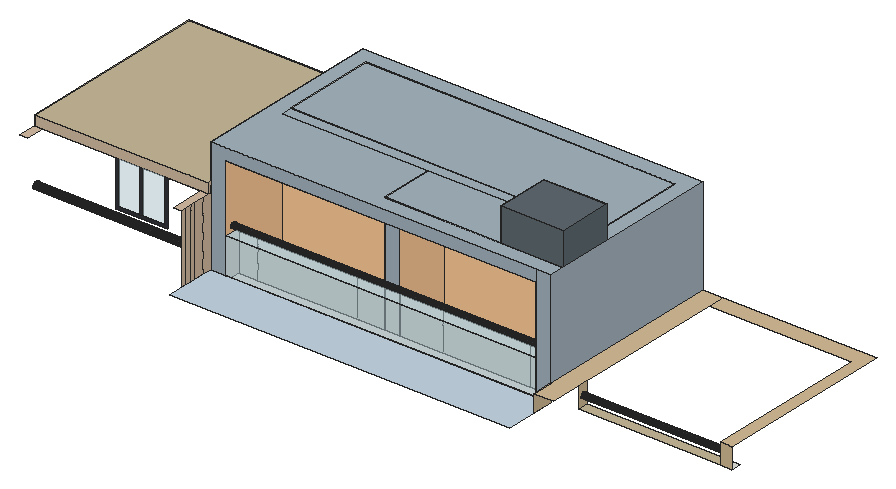
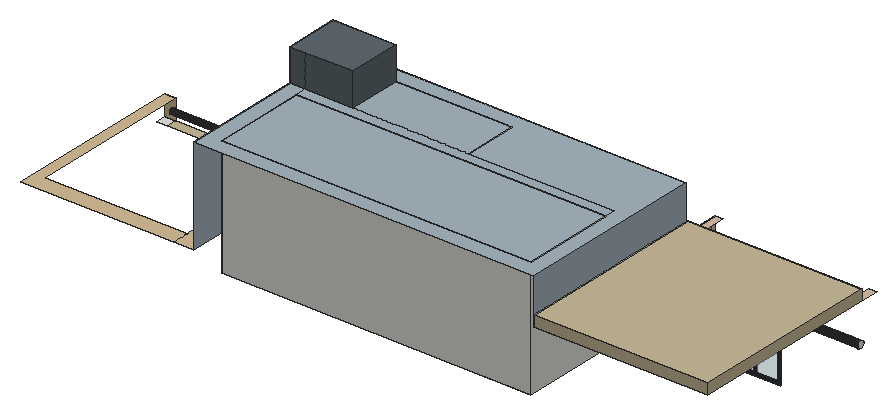
# SketchUp Ruby script. Lengths in inches.
U = 1.inch
M = Sketchup.active_model
def pt(a) = Geom::Point3d.new(a.map { |v| v * U })
def face(e, loops, mat)
  f = e.add_face(loops[0].map { |a| pt(a) })
  loops[1..].each { |l| e.add_face(l.map { |a| pt(a) }).erase! }
  f.material = f.back_material = mat if mat
  f
end
# faces: each face lists its corners as indices into pts; further lists are holes
def faces(e, pts, list, mat = nil) = list.each { |f| face(e, (f[0].is_a?(Array) ? f : [f]).map { |l| l.map { |i| pts[i] } }, mat) }
# xy, xz, yz: faces in a plane at the given z, y or x. An outline is a flat list of corners, or four numbers for a rectangle; further outlines are holes
def ring(l) = l.size == 4 ? [[l[0], l[1]], [l[2], l[1]], [l[2], l[3]], [l[0], l[3]]] : l.each_slice(2).to_a
def flat(e, list, mat, &to3) = list.each { |f| face(e, (f[0].is_a?(Array) ? f : [f]).map { |l| ring(l).map { |u, v| to3.(u, v) } }, mat) }
def xy(e, z, list, mat = nil) = flat(e, list, mat) { |x, y| [x, y, z] }
def xz(e, y, list, mat = nil) = flat(e, list, mat) { |x, z| [x, y, z] }
def yz(e, x, list, mat = nil) = flat(e, list, mat) { |y, z| [x, y, z] }
def lines(e, pts, list) = list.each { |a, b| e.add_line(pt(pts[a]), pt(pts[b])) }
# prism: a flat outline (further loops are holes) pulled along v
def prism(e, loops, v, mat = nil)
  f = face(e, loops, mat); d = Geom::Vector3d.new(v.map { |x| x * U })
  f.pushpull(f.normal.samedirection?(d) ? d.length : -d.length)
end
def box(e, o, s, mat = nil) = prism(e, [[o, [o[0] + s[0], o[1], o[2]], [o[0] + s[0], o[1] + s[1], o[2]], [o[0], o[1] + s[1], o[2]]]], [0, 0, s[2]], mat)
def at(x, y, z, deg = 0) = Geom::Transformation.translation(pt([x, y, z])) * Geom::Transformation.rotation(ORIGIN, Z_AXIS, deg.degrees)
def axes(o, x, y, z) = Geom::Transformation.new([*x, 0, *y, 0, *z, 0, *pt(o).to_a, 1])
def part(name) = M.definitions.add(name)
# library, detail: a bought-in or finely detailed component or shape, given as its bounding box
def library(name, o, s) = part(name).tap { |d| box(d.entities, o, s) }
def detail(e, o, s) = box(e.add_group.entities, o, s)
def put(e, d, t, mat = nil) = e.add_instance(d, t).tap { |i| i.material = mat if mat }
def group(e, t, mat = nil) = e.add_group.tap { |g| g.transformation = t; g.material = mat if mat }.entities
root = M.entities
M.materials.add("[Color C02]").color = [255, 204, 153]
M.materials.add("[Formica Beige]").color = [211, 187, 149]
M.materials.add("[Formica Laminate Dark]").color = [50, 53, 60]
M.materials.add("[Formica Laminate Light]").color = [213, 189, 164]
M.materials.add("[Formica Speckled Grey]").color = [94, 105, 111]
M.materials.add("[Quartz Light Brown]").color = [199, 184, 152]
M.materials.add("[Terrazzo Light Blue]1").color = [165, 180, 191]
M.materials.add("[Terrazzo Light Blue]2").color = [196, 214, 227]
M.materials.add("[Translucent Glass Safety]").color = [204, 235, 244]
M.materials["[Translucent Glass Safety]"].alpha = 0.5
xy(root,657,[[216.23,147.05,570.64,164.71],[216.23,164.71,383.2,226.73],[401.21,164.71,570.64,226.73],[216.23,239.39,570.64,346.47]])
xy(root,658.875,[[774.15,157.7,786.87,169.39]])
xy(root,658.875,[[611.125,157.7,774.15,169.39]],"[Quartz Light Brown]")
xy(root,662.0625,[[198.57,88.2,588.3,147.05]],"[Terrazzo Light Blue]2")
xy(root,682.5,[[588.3,122.79,611.125,364.125],[774.15,157.7,786.87,157.7,786.87,364.125,611.125,364.125,611.125,344.36,774.15,344.36]],"[Formica Beige]")
xy(root,686.625,[[60.55,130.88,61.23,130.97,61.87,131.23,62.41,131.65,62.83,132.19,63.09,132.82,63.18,133.5,63.09,134.18,62.83,134.81,62.41,135.36,61.87,135.78,61.23,136.04,60.55,136.13,59.875,136.04,59.24,135.78,58.7,135.36,58.28,134.81,58.02,134.18,57.93,133.5,58.02,132.82,58.28,132.19,58.7,131.65,59.24,131.23,59.875,130.97]])
xy(root,687.6875,[[117.43,130.88,118.11,130.97,118.74,131.23,119.28,131.65,119.7,132.19,119.96,132.82,120.05,133.5,119.96,134.18,119.7,134.81,119.28,135.36,118.74,135.78,118.11,136.04,117.43,136.13,116.75,136.04,116.12,135.78,115.57,135.36,115.15,134.81,114.89,134.18,114.8,133.5,114.89,132.82,115.15,132.19,115.57,131.65,116.12,131.23,116.75,130.97]])
xy(root,688.0625,[[140.74,130.88,141.42,130.97,142.05,131.23,142.6,131.65,143.01,132.19,143.28,132.82,143.37,133.5,143.28,134.18,143.01,134.81,142.6,135.36,142.05,135.78,141.42,136.04,140.74,136.13,140.0625,136.04,139.43,135.78,138.88,135.36,138.47,134.81,138.2,134.18,138.12,133.5,138.2,132.82,138.47,132.19,138.88,131.65,139.43,131.23,140.0625,130.97]])
xy(root,688.5,[[179.99,130.88,180.67,130.97,181.3,131.23,181.85,131.65,182.26,132.19,182.53,132.82,182.62,133.5,182.53,134.18,182.26,134.81,181.85,135.36,181.3,135.78,180.67,136.04,179.99,136.13,179.3125,136.04,178.68,135.78,178.13,135.36,177.72,134.81,177.45,134.18,177.37,133.5,177.45,132.82,177.72,132.19,178.13,131.65,178.68,131.23,179.3125,130.97]])
xy(root,688.68,[[161.99,130.88,162.67,130.97,163.3,131.23,163.85,131.65,164.26,132.19,164.53,132.82,164.62,133.5,164.53,134.18,164.26,134.81,163.85,135.36,163.3,135.78,162.67,136.04,161.99,136.13,161.3125,136.04,160.68,135.78,160.13,135.36,159.72,134.81,159.45,134.18,159.37,133.5,159.45,132.82,159.72,132.19,160.13,131.65,160.68,131.23,161.3125,130.97]])
xy(root,688.6875,[[94.37,130.88,95.04,130.97,95.68,131.23,96.22,131.65,96.64,132.19,96.9,132.82,96.99,133.5,96.9,134.18,96.64,134.81,96.22,135.36,95.68,135.78,95.04,136.04,94.37,136.13,93.6875,136.04,93.05,135.78,92.51,135.36,92.09,134.81,91.83,134.18,91.74,133.5,91.83,132.82,92.09,132.19,92.51,131.65,93.05,131.23,93.6875,130.97]])
xy(root,689.58,[[41.37,130.88,42.04,130.97,42.68,131.23,43.22,131.65,43.64,132.19,43.9,132.82,43.99,133.5,43.9,134.18,43.64,134.81,43.22,135.36,42.68,135.78,42.04,136.04,41.37,136.13,40.6875,136.04,40.05,135.78,39.51,135.36,39.09,134.81,38.83,134.18,38.74,133.5,38.83,132.82,39.09,132.19,39.51,131.65,40.05,131.23,40.6875,130.97],[75.99,130.88,76.67,130.97,77.3,131.23,77.85,131.65,78.26,132.19,78.53,132.82,78.62,133.5,78.53,134.18,78.26,134.81,77.85,135.36,77.3,135.78,76.67,136.04,75.99,136.13,75.3125,136.04,74.68,135.78,74.13,135.36,73.72,134.81,73.45,134.18,73.37,133.5,73.45,132.82,73.72,132.19,74.13,131.65,74.68,131.23,75.3125,130.97]])
xy(root,690.36,[[23.62,130.88,24.29,130.97,24.93,131.23,25.47,131.65,25.89,132.19,26.15,132.82,26.24,133.5,26.15,134.18,25.89,134.81,25.47,135.36,24.93,135.78,24.29,136.04,23.62,136.13,22.9375,136.04,22.3,135.78,21.76,135.36,21.34,134.81,21.08,134.18,20.99,133.5,21.08,132.82,21.34,132.19,21.76,131.65,22.3,131.23,22.9375,130.97]])
xy(root,702.25,[[216.23,147.05,570.64,164.71]],"[Translucent Glass Safety]")
xy(root,721.83,[[46.64,183.96,124.14,191.15]],"[Formica Beige]")
xy(root,726.77,[[46.64,183.96,124.14,191.15]],"[Formica Beige]")
xy(root,740.5625,[[0,144.21,0,364.125,198.57,364.125,198.57,144.21,189.57,144.21,189.57,191.15,9,191.15,9,144.21]])
xy(root,740.5625,[[9,144.21,189.57,191.15]],"[Formica Beige]")
xy(root,740.5625,[[189.57,105.54,198.57,144.21],[0,122.79,9,144.21]],"[Formica Laminate Light]")
xy(root,752.5625,[[0,144.21,198.57,364.125]],"[Quartz Light Brown]")
xy(root,779.88,[[216.23,147.05,216.23,226.73,383.2,226.73,383.2,164.71,570.64,164.71,570.64,147.05],[401.21,164.71,570.64,226.73]],"[Formica Beige]")
xy(root,793.1875,[[515.97,164.71,588.3,226.73]])
xy(root,793.1875,[[198.57,147.05,588.3,147.05,588.3,164.71,383.2,164.71,383.2,226.73,216.23,226.73,216.23,346.47,570.64,346.47,570.64,226.73,588.3,226.73,588.3,364.125,198.57,364.125],[383.2,164.71,515.97,226.73],[216.23,226.73,570.64,239.39],[216.23,239.39,570.64,346.47]],"[Terrazzo Light Blue]1")
xy(root,830.875,[[515.97,164.71,588.3,226.73]],"[Formica Speckled Grey]")
xz(root,144.21,[[0,740.5625,198.57,752.5625]],"[Formica Laminate Light]")
xz(root,147.05,[[216.23,657,570.64,662.0625]])
xz(root,147.05,[[198.57,662.0625,216.23,662.0625,216.23,779.88,570.64,779.88,570.64,793.1875,198.57,793.1875],[570.64,662.0625,588.3,793.1875]],"[Terrazzo Light Blue]1")
xz(root,147.05,[[216.23,662.0625,570.64,702.25]],"[Translucent Glass Safety]")
xz(root,157.7,[[774.15,658.875,786.87,682.5]],"[Formica Beige]")
xz(root,164.71,[[216.23,657,238.58,702.25],[238.58,657,351.88,702.25],[351.88,657,383.2,702.25],[383.2,657,401.21,702.25],[401.21,657,450.54,702.25],
  [450.54,657,549.2,702.25],[549.2,657,570.64,702.25],[383.2,779.88,570.64,793.1875]])
xz(root,164.71,[[515.97,793.1875,588.3,830.875]],"[Formica Speckled Grey]")
xz(root,164.71,[[383.2,702.25,401.21,779.88]],"[Terrazzo Light Blue]1")
xz(root,183.96,[[46.64,721.83,124.14,726.77]],"[Formica Beige]")
xz(root,191.15,[[[54.875,654.41,114.625,720.78],[58.53,658.07,110.97,717.13]],[81.875,658.07,85.9,717.13]],"[Formica Laminate Dark]")
xz(root,191.15,[[58.53,658.07,81.875,717.13],[85.9,658.07,110.97,717.13]],"[Translucent Glass Safety]")
xz(root,226.73,[[216.23,657,383.2,779.88],[401.21,657,570.64,779.88]],"[Color C02]")
xz(root,226.73,[[515.97,793.1875,570.64,830.875],[570.64,793.1875,588.3,830.875]],"[Formica Speckled Grey]")
xz(root,239.39,[[216.23,657,570.64,793.1875]])
xz(root,346.47,[[216.23,657,570.64,793.1875]])
xz(root,364.125,[[0,740.5625,198.57,752.5625]],"[Quartz Light Brown]")
yz(root,0,[[144.21,740.5625,364.125,752.5625]],"[Quartz Light Brown]")
yz(root,9,[[133.5,683.96,132.53,684.08,131.63,684.46,130.85,685.06,130.25,685.83,129.88,686.74,129.75,687.71,129.88,688.68,130.25,689.58,130.85,690.36,131.63,690.95,132.53,691.33,133.5,691.46,134.47,691.33,135.38,690.95,136.15,690.36,136.75,689.58,137.125,688.68,137.25,687.71,137.125,686.74,136.75,685.83,136.15,685.06,135.38,684.46,134.47,684.08]])
yz(root,46.64,[[183.96,721.83,191.15,726.77]],"[Formica Beige]")
yz(root,124.14,[[183.96,721.83,191.15,726.77]],"[Formica Beige]")
yz(root,198.57,[[147.05,740.5625,364.125,752.5625]])
yz(root,198.57,[[105.54,662.0625,110.07,740.5625],[110.07,662.0625,119.07,740.5625],[119.07,662.0625,122.79,740.5625],[122.79,662.0625,135.71,740.5625],[135.71,662.0625,147.05,740.5625],
  [144.21,740.5625,147.05,752.5625]],"[Formica Laminate Light]")
yz(root,198.57,[[147.05,752.5625,364.125,793.1875]],"[Terrazzo Light Blue]1")
yz(root,216.23,[[147.05,657,164.71,702.25],[239.39,657,346.47,793.1875]])
yz(root,216.23,[[[164.71,657,226.73,657,226.73,779.88,147.05,779.88,147.05,702.25,164.71,702.25],[155.88,707.26,155.11,707.36,154.38,707.66,153.76,708.13,153.28,708.76,152.99,709.48,152.88,710.26,152.99,711.03,153.28,711.76,153.76,712.375,154.38,712.85,155.11,713.15,155.88,713.26,156.66,713.15,157.38,712.85,158,712.375,158.48,711.76,158.78,711.03,158.88,710.26,158.78,709.48,158.48,708.76,158,708.13,157.38,707.66,156.66,707.36]]],"[Color C02]")
yz(root,383.2,[[164.71,779.88,226.73,793.1875]])
yz(root,383.2,[[164.71,657,226.73,779.88]],"[Color C02]")
yz(root,401.21,[[164.71,657,226.73,779.88]],"[Color C02]")
yz(root,515.97,[[164.71,793.1875,226.73,830.875]],"[Formica Speckled Grey]")
yz(root,570.64,[[147.05,657,164.71,702.25],[239.39,657,346.47,793.1875],[155.88,707.26,156.66,707.36,157.38,707.66,158,708.13,158.48,708.76,158.78,709.48,158.88,710.26,158.78,711.03,158.48,711.76,158,712.375,157.38,712.85,156.66,713.15,155.88,713.26,155.11,713.15,154.38,712.85,153.76,712.375,153.28,711.76,152.99,711.03,152.88,710.26,152.99,709.48,153.28,708.76,153.76,708.13,154.38,707.66,155.11,707.36]])
yz(root,570.64,[[[164.71,657,164.71,702.25,147.05,702.25,147.05,779.88,226.73,779.88,226.73,657],[155.88,707.26,156.66,707.36,157.38,707.66,158,708.13,158.48,708.76,158.78,709.48,158.88,710.26,158.78,711.03,158.48,711.76,158,712.375,157.38,712.85,156.66,713.15,155.88,713.26,155.11,713.15,154.38,712.85,153.76,712.375,153.28,711.76,152.99,711.03,152.88,710.26,152.99,709.48,153.28,708.76,153.76,708.13,154.38,707.66,155.11,707.36]]],"[Color C02]")
yz(root,588.3,[[122.79,662.0625,147.05,682.5]],"[Formica Beige]")
yz(root,588.3,[[164.71,793.1875,226.73,830.875]],"[Formica Speckled Grey]")
yz(root,588.3,[[147.05,682.5,364.125,793.1875]],"[Terrazzo Light Blue]1")
yz(root,611.125,[[163.52,668.49,162.76,668.59,162.06,668.89,161.45,669.35,160.98,669.96,160.6875,670.67,160.59,671.43,160.6875,672.19,160.98,672.9,161.45,673.51,162.06,673.97,162.76,674.27,163.52,674.37,164.28,674.27,164.99,673.97,165.6,673.51,166.07,672.9,166.36,672.19,166.46,671.43,166.36,670.67,166.07,669.96,165.6,669.35,164.99,668.89,164.28,668.59]])
yz(root,611.125,[[[157.7,658.875,169.39,682.5],[163.52,668.49,162.76,668.59,162.06,668.89,161.45,669.35,160.98,669.96,160.6875,670.67,160.59,671.43,160.6875,672.19,160.98,672.9,161.45,673.51,162.06,673.97,162.76,674.27,163.52,674.37,164.28,674.27,164.99,673.97,165.6,673.51,166.07,672.9,166.36,672.19,166.46,671.43,166.36,670.67,166.07,669.96,165.6,669.35,164.99,668.89,164.28,668.59]]],"[Formica Beige]")
p = [[611.125,162.76,668.59],[611.125,163.52,668.49],[774.15,163.52,668.49],[774.15,162.76,668.59],[611.125,164.28,668.59],[774.15,164.28,668.59],
  [611.125,162.06,668.89],[774.15,162.06,668.89],[611.125,164.99,668.89],[774.15,164.99,668.89],[611.125,161.45,669.35],[774.15,161.45,669.35],
  [611.125,165.6,669.35],[774.15,165.6,669.35],[611.125,160.98,669.96],[774.15,160.98,669.96],[611.125,166.07,669.96],[774.15,166.07,669.96],
  [611.125,160.6875,670.67],[774.15,160.6875,670.67],[611.125,166.36,670.67],[774.15,166.36,670.67],[611.125,160.59,671.43],[774.15,160.59,671.43],
  [611.125,166.46,671.43],[774.15,166.46,671.43],[611.125,160.6875,672.19],[774.15,160.6875,672.19],[611.125,166.36,672.19],[774.15,166.36,672.19],
  [611.125,160.98,672.9],[774.15,160.98,672.9],[611.125,166.07,672.9],[774.15,166.07,672.9],[611.125,161.45,673.51],[774.15,161.45,673.51],
  [611.125,165.6,673.51],[774.15,165.6,673.51],[611.125,162.06,673.97],[774.15,162.06,673.97],[611.125,164.99,673.97],[774.15,164.99,673.97],
  [611.125,162.76,674.27],[774.15,162.76,674.27],[611.125,164.28,674.27],[774.15,164.28,674.27],[611.125,163.52,674.37],[774.15,163.52,674.37],
  [9,132.53,684.08],[9,133.5,683.96],[20.99,133.5,683.96],[26.24,133.5,683.96],[38.74,133.5,683.96],[43.99,133.5,683.96],
  [57.93,133.5,683.96],[63.18,133.5,683.96],[73.37,133.5,683.96],[78.62,133.5,683.96],[91.74,133.5,683.96],[96.99,133.5,683.96],
  [114.8,133.5,683.96],[120.05,133.5,683.96],[138.12,133.5,683.96],[143.37,133.5,683.96],[159.37,133.5,683.96],[164.62,133.5,683.96],
  [177.37,133.5,683.96],[182.62,133.5,683.96],[189.57,133.5,683.96],[189.57,132.53,684.08],[9,134.47,684.08],[189.57,134.47,684.08],
  [9,131.63,684.46],[189.57,131.63,684.46],[9,135.38,684.46],[189.57,135.38,684.46],[9,130.85,685.06],[189.57,130.85,685.06],
  [9,136.15,685.06],[189.57,136.15,685.06],[9,130.25,685.83],[189.57,130.25,685.83],[9,136.75,685.83],[189.57,136.75,685.83],
  [9,129.88,686.74],[189.57,129.88,686.74],[9,137.125,686.74],[189.57,137.125,686.74],[9,129.75,687.71],[189.57,129.75,687.71],
  [9,137.25,687.71],[189.57,137.25,687.71],[9,129.88,688.68],[189.57,129.88,688.68],[9,137.125,688.68],[189.57,137.125,688.68],
  [9,130.25,689.58],[189.57,130.25,689.58],[9,136.75,689.58],[189.57,136.75,689.58],[9,130.85,690.36],[189.57,130.85,690.36],
  [9,136.15,690.36],[189.57,136.15,690.36],[9,131.63,690.95],[189.57,131.63,690.95],[9,135.38,690.95],[189.57,135.38,690.95],
  [9,132.53,691.33],[189.57,132.53,691.33],[9,134.47,691.33],[189.57,134.47,691.33],[9,133.5,691.46],[189.57,133.5,691.46],
  [570.64,155.88,707.26],[570.64,155.11,707.36],[216.23,155.11,707.36],[216.23,155.88,707.26],[570.64,156.66,707.36],[216.23,156.66,707.36],
  [570.64,154.38,707.66],[216.23,154.38,707.66],[570.64,157.38,707.66],[216.23,157.38,707.66],[570.64,153.76,708.13],[216.23,153.76,708.13],
  [570.64,158,708.13],[216.23,158,708.13],[570.64,153.28,708.76],[216.23,153.28,708.76],[570.64,158.48,708.76],[216.23,158.48,708.76],
  [570.64,152.99,709.48],[216.23,152.99,709.48],[570.64,158.78,709.48],[216.23,158.78,709.48],[570.64,152.88,710.26],[216.23,152.88,710.26],
  [570.64,158.88,710.26],[216.23,158.88,710.26],[570.64,152.99,711.03],[216.23,152.99,711.03],[570.64,158.78,711.03],[216.23,158.78,711.03],
  [570.64,153.28,711.76],[216.23,153.28,711.76],[570.64,158.48,711.76],[216.23,158.48,711.76],[570.64,153.76,712.375],[216.23,153.76,712.375],
  [570.64,158,712.375],[216.23,158,712.375],[570.64,154.38,712.85],[216.23,154.38,712.85],[570.64,157.38,712.85],[216.23,157.38,712.85],
  [570.64,155.11,713.15],[216.23,155.11,713.15],[570.64,156.66,713.15],[216.23,156.66,713.15],[570.64,155.88,713.26],[216.23,155.88,713.26]]
faces(root,p,[[0,1,2,3],[1,4,5,2],[6,0,3,7],[4,8,9,5],[10,6,7,11],[8,12,13,9],[14,10,11,15],[12,16,17,13],
  [18,14,15,19],[16,20,21,17],[22,18,19,23],[20,24,25,21],[26,22,23,27],[24,28,29,25],[30,26,27,31],[28,32,33,29],
  [34,30,31,35],[32,36,37,33],[38,34,35,39],[36,40,41,37],[42,38,39,43],[40,44,45,41],[46,42,43,47],[44,46,47,45],
  [48,49,50,51,52,53,54,55,56,57,58,59,60,61,62,63,64,65,66,67,68,69],[49,70,71,68,67,66,65,64,63,62,61,60,59,58,57,56,55,54,53,52,51,50],[72,48,69,73],[70,74,75,71],[76,72,73,77],[74,78,79,75],[80,76,77,81],[78,82,83,79],
  [84,80,81,85],[82,86,87,83],[88,84,85,89],[86,90,91,87],[92,88,89,93],[90,94,95,91],[96,92,93,97],[94,98,99,95],
  [100,96,97,101],[98,102,103,99],[104,100,101,105],[102,106,107,103],[108,104,105,109],[106,110,111,107],[112,108,109,113],[110,112,113,111],
  [114,115,116,117],[118,114,117,119],[115,120,121,116],[122,118,119,123],[120,124,125,121],[126,122,123,127],[124,128,129,125],[130,126,127,131],
  [128,132,133,129],[134,130,131,135],[132,136,137,133],[138,134,135,139],[136,140,141,137],[142,138,139,143],[140,144,145,141],[146,142,143,147],
  [144,148,149,145],[150,146,147,151],[148,152,153,149],[154,150,151,155],[152,156,157,153],[158,154,155,159],[156,160,161,157],[160,158,159,161]],"[Formica Laminate Dark]")
